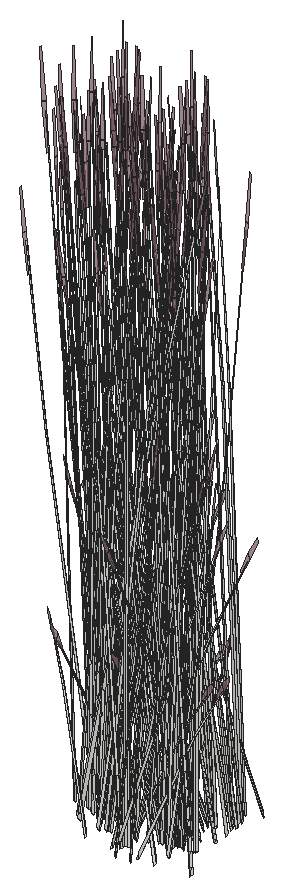
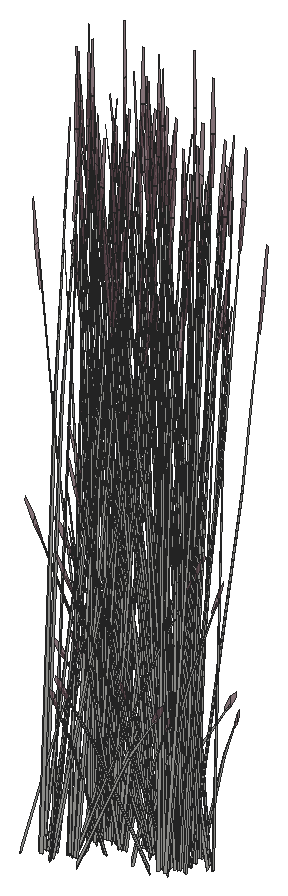
# SketchUp Ruby script. Lengths in inches.
U = 1.inch
M = Sketchup.active_model
def pt(a) = Geom::Point3d.new(a.map { |v| v * U })
def face(e, loops, mat)
  f = e.add_face(loops[0].map { |a| pt(a) })
  loops[1..].each { |l| e.add_face(l.map { |a| pt(a) }).erase! }
  f.material = f.back_material = mat if mat
  f
end
# faces: each face lists its corners as indices into pts; further lists are holes
def faces(e, pts, list, mat = nil) = list.each { |f| face(e, (f[0].is_a?(Array) ? f : [f]).map { |l| l.map { |i| pts[i] } }, mat) }
# xy, xz, yz: faces in a plane at the given z, y or x. An outline is a flat list of corners, or four numbers for a rectangle; further outlines are holes
def ring(l) = l.size == 4 ? [[l[0], l[1]], [l[2], l[1]], [l[2], l[3]], [l[0], l[3]]] : l.each_slice(2).to_a
def flat(e, list, mat, &to3) = list.each { |f| face(e, (f[0].is_a?(Array) ? f : [f]).map { |l| ring(l).map { |u, v| to3.(u, v) } }, mat) }
def xy(e, z, list, mat = nil) = flat(e, list, mat) { |x, y| [x, y, z] }
def xz(e, y, list, mat = nil) = flat(e, list, mat) { |x, z| [x, y, z] }
def yz(e, x, list, mat = nil) = flat(e, list, mat) { |y, z| [x, y, z] }
def lines(e, pts, list) = list.each { |a, b| e.add_line(pt(pts[a]), pt(pts[b])) }
# prism: a flat outline (further loops are holes) pulled along v
def prism(e, loops, v, mat = nil)
  f = face(e, loops, mat); d = Geom::Vector3d.new(v.map { |x| x * U })
  f.pushpull(f.normal.samedirection?(d) ? d.length : -d.length)
end
def box(e, o, s, mat = nil) = prism(e, [[o, [o[0] + s[0], o[1], o[2]], [o[0] + s[0], o[1] + s[1], o[2]], [o[0], o[1] + s[1], o[2]]]], [0, 0, s[2]], mat)
def at(x, y, z, deg = 0) = Geom::Transformation.translation(pt([x, y, z])) * Geom::Transformation.rotation(ORIGIN, Z_AXIS, deg.degrees)
def axes(o, x, y, z) = Geom::Transformation.new([*x, 0, *y, 0, *z, 0, *pt(o).to_a, 1])
def part(name) = M.definitions.add(name)
# library, detail: a bought-in or finely detailed component or shape, given as its bounding box
def library(name, o, s) = part(name).tap { |d| box(d.entities, o, s) }
def detail(e, o, s) = box(e.add_group.entities, o, s)
def put(e, d, t, mat = nil) = e.add_instance(d, t).tap { |i| i.material = mat if mat }
def group(e, t, mat = nil) = e.add_group.tap { |g| g.transformation = t; g.material = mat if mat }.entities
root = M.entities
M.materials.add("LightPink_Translucent").color = [144, 107, 117]
M.materials["LightPink_Translucent"].alpha = 0.75
c1 = part("blade")
p = [[2.15,0.21,22],[0,0.17,0],[0.09,0.45,0],[2.18,0.31,22],[2.29,0.31,22],[0.38,0.45,0],
  [2.48,0.24,33],[2.49,0.24,33],[2.48,0.22,33]]
faces(c1.entities,p,[[0,1,2,3],[4,5,2,3],[6,3,4,7],[8,0,3,6]])
c2 = part("seeds")
p = [[0.3,-0.1,1.38],[-0.01,-0.03,1.59],[-0.01,-0.03,0.03],[0.14,-0.07,-0.07],[0.29,-0.03,3],[0.15,0.01,3.11]]
faces(c2.entities,p,[[0,1,2,3],[1,0,4,5]],"LightPink_Translucent")
c3 = part("blade with seeds")
put(c3.entities,c1,at(0,0,0))
put(c3.entities,c2,axes([2.4,0.25,30.99],[1.5799,-0.05474,1.17369],[-0.12525,1.92788,0.29478],[-0.07173,-0.02425,1.56792]))
put(root,c3,axes([329.37,18.01,50.06],[0.63212,0.12701,0.27176],[-0.15814,0.45398,-0.32244],[-0.10462,0.05682,1.45692]))
put(root,c3,axes([329.32,18.31,49.78],[-0.47255,0.19538,-0.43871],[-0.28245,-0.35034,0],[-0.10763,0.0445,1.3917]))
put(root,c3,axes([334.98,18.31,49.78],[-0.47255,0.19538,-0.43871],[-0.28245,-0.35034,0],[-0.10763,0.0445,1.3917]))
put(root,c3,axes([330.85,20.33,50.4],[-0.24498,0.3521,0.39531],[-0.50902,-0.16945,-0.19025],[0,-0.08116,1.26923]))
put(root,c3,axes([330.89,17.16,49.78],[0,0.39075,-0.43871],[-0.56491,0,0],[0,0.089,1.3917]))
put(root,c3,axes([325.16,20.15,50.4],[-0.54829,0.02412,0.39531],[-0.04958,-0.40041,-0.19025],[0.09816,-0.04058,1.26923]))
put(root,c3,axes([331.75,20.02,49.95],[0,-0.45213,0],[0.63136,0,0],[0,0,1.58567]))
put(root,c3,axes([323.75,20.4375,50.19],[0,0.39075,0.43871],[-0.56491,0,0],[0,-0.089,1.3917]))
put(root,c3,axes([326.97,19.08,50.1],[0.31568,-0.39156,0],[0.52815,0.21836,-0.456],[0.12029,0.04973,1.44655]))
put(root,c3,axes([325.08,20.75,49.95],[-0.30332,-0.32798,-0.39531],[0.45944,-0.23096,0.19025],[-0.09816,-0.04058,1.26923]))
put(root,c3,axes([325.14,20.29,50.09],[0.21952,0.43694,0.40429],[-0.62724,0.15194,0.15865],[0.00767,-0.08029,1.40366]))
put(root,c3,axes([330.625,20.57,49.82],[-0.52523,-0.06406,-0.55095],[0.11084,-0.39517,-0.1446],[-0.15674,-0.04788,1.21613]))
put(root,c3,axes([331.45,19.74,50.09],[-0.41865,0.35461,0.40429],[-0.49737,-0.31303,0.15865],[0.10093,-0.03539,1.40366]))
put(root,c3,axes([328.21,20.625,49.75],[-0.3252,0.04689,1.25103],[-0.05176,-0.37326,0.07161],[0.22777,-0.0565,0.71188]))
put(root,c3,axes([328.8,20.3,50],[-0.31304,-0.24986,-0.05733],[0.34284,-0.22894,-0.25992],[0.09714,-0.01612,0.85731]))
put(root,c3,axes([331.91,20.37,50.03],[-0.46965,-0.33633,-0.05417],[0.46994,-0.33653,0],[-0.0164,-0.01174,1.55135]))
put(root,c3,axes([332.55,22.4,50.29],[-0.03058,0.12783,1.26356],[-0.44698,0.10701,-0.27174],[-0.10448,-0.16522,0.54024]))
put(root,c3,axes([325.03,20.64,50.4],[-0.24498,0.3521,0.39531],[-0.50902,-0.16945,-0.19025],[0,-0.08116,1.26923]))
put(root,c3,axes([330.72,19.15,50.1875],[-0.14586,0.38834,0.15589],[-0.53375,-0.1099,0.31002],[0.0922,-0.00189,1.41735]))
put(root,c3,axes([325.93,20.33,49.95],[0,-0.45213,0],[0.63136,0,0],[0,0,1.58567]))
put(root,c3,axes([326.7,19.28,50.19],[-0.47255,-0.19538,0.43871],[0.28245,-0.35034,0],[0.10763,0.0445,1.3917]))
put(root,c3,axes([329.75,18.25,50.1],[0.31568,0.39156,0],[-0.52815,0.21836,-0.456],[-0.12029,0.04973,1.44655]))
put(root,c3,axes([331.01,20.41,50.09],[0.63817,0.08233,0.40429],[-0.12987,0.46497,0.15865],[-0.09326,-0.0449,1.40366]))
put(root,c3,axes([330.25,18.39,49.32],[0.03679,-0.05641,1.55816],[0.46313,-0.16615,-0.23804],[0.14041,0.08599,0.26541]))
put(root,c3,axes([329.64,17.1,49.85],[0.18514,0.35777,-0.61156],[-0.53331,0.12885,-0.16051],[0.02046,0.12115,1.3499]))
put(root,c3,axes([325.63,20.04,50.09],[-0.41865,0.35461,0.40429],[-0.49737,-0.31303,0.15865],[0.10093,-0.03539,1.40366]))
put(root,c3,axes([326,18.34,49.32],[0.06773,0.03904,1.55816],[0.11484,0.36171,-0.23804],[-0.15011,0.07713,0.26541]))
put(root,c3,axes([331.66,18.34,49.32],[0.06773,0.03904,1.55816],[0.11484,0.36171,-0.23804],[-0.15011,0.07713,0.26541]))
put(root,c3,axes([328.94,20.01,49.32],[0.0128,0.06158,1.55816],[-0.25814,0.3216,-0.23804],[-0.18336,-0.01621,0.26541]))
put(root,c3,axes([331.63,19.68,50.4],[-0.30332,-0.32798,0.39531],[0.45944,-0.23096,-0.19025],[0.09816,0.04058,1.26923]))
put(root,c3,axes([326.09,20.68,50.03],[-0.46965,-0.33633,-0.05417],[0.46994,-0.33653,0],[-0.0164,-0.01174,1.55135]))
put(root,c3,axes([330.07,21.17,49.79],[-0.11861,-0.34048,-0.27372],[0.47106,-0.09668,0.27372],[-0.09497,-0.03926,1.22797]))
put(root,c3,axes([324.91,19.46,50.1875],[-0.14586,0.38834,0.15589],[-0.53375,-0.1099,0.31002],[0.0922,-0.00189,1.41735]))
put(root,c3,axes([324.68,19.77,49.41],[-0.49699,0.15644,1.13921],[-0.15819,-0.44887,0.44265],[0.30518,0.00747,1.29573]))
put(root,c3,axes([326.02,19.89,50.3125],[0.09741,-0.34873,0.12794],[0.4759,0.06053,-0.36534],[0.08661,0.03581,1.11991]))
put(root,c3,axes([330.67,21.15,50.1875],[0.54257,-0.10371,0.15589],[0.13397,0.38597,0.31002],[-0.04839,-0.05624,1.41735]))
put(root,c3,axes([330.22,18.48,50.36],[-0.32378,-0.01225,0.92831],[0.21383,-0.26028,0.51254],[0.12791,0.09247,0.72818]))
put(root,c3,axes([325.2,20.72,50.09],[0.63817,0.08233,0.40429],[-0.12987,0.46497,0.15865],[-0.09326,-0.0449,1.40366]))
put(root,c3,axes([328.57,20.38,49.32],[-0.02639,-0.05932,1.55816],[0.18302,-0.34702,-0.23804],[0.18462,-0.00499,0.26541]))
put(root,c3,axes([329.93,21.32,49.78],[-0.47255,-0.19538,-0.43871],[0.28245,-0.35034,0],[-0.10763,-0.0445,1.3917]))
put(root,c3,axes([325.82,19.98,50.4],[-0.30332,-0.32798,0.39531],[0.45944,-0.23096,-0.19025],[0.09816,0.04058,1.26923]))
put(root,c3,axes([332.18,20.12,49.95],[0.56491,0,0],[0,0.40454,0],[0,0,1.5764]))
put(root,c3,axes([331.22,20.63,50.36],[-0.50979,0.25942,-0.25709],[-0.339,-0.36656,-0.44182],[-0.12578,-0.03723,1.41118]))
put(root,c3,axes([332.34,19.17,50.1875],[-0.54257,0.10371,0.15589],[-0.13397,-0.38597,0.31002],[0.04839,0.05624,1.41735]))
put(root,c3,axes([324.85,21.46,50.1875],[0.54257,-0.10371,0.15589],[0.13397,0.38597,0.31002],[-0.04839,-0.05624,1.41735]))
put(root,c3,axes([325.97,20,50.36],[0.50979,-0.25942,-0.25709],[0.339,0.36656,-0.44182],[0.12578,0.03723,1.41118]))
put(root,c3,axes([329.16,17.85,50.29],[0.00891,-0.12953,1.26356],[0.4258,-0.14469,-0.27174],[0.13144,0.15503,0.54024]))
put(root,c3,axes([327.26,19.31,49.78],[0.47255,0.19538,-0.43871],[-0.28245,0.35034,0],[0.10763,0.0445,1.3917]))
put(root,c3,axes([326.36,20.43,49.95],[0.56491,0,0],[0,0.40454,0],[0,0,1.5764]))
put(root,c3,axes([331.99,19.92,50.1],[-0.63817,-0.08233,0.43472],[0.12987,-0.46497,0.17059],[0.09326,0.0449,1.50931]))
put(root,c3,axes([331.49,21.0625,49.95],[-0.16474,-0.33688,0],[0.47043,-0.11798,0],[0,0,1.36402]))
put(root,c3,axes([326.52,19.48,50.1875],[-0.54257,0.10371,0.15589],[-0.13397,-0.38597,0.31002],[0.04839,0.05624,1.41735]))
put(root,c3,axes([331.17,20.74,50.3125],[-0.09741,0.34873,0.12794],[-0.4759,-0.06053,-0.36534],[-0.08661,-0.03581,1.11991]))
put(root,c3,axes([332.29,21.18,50.1875],[0.14586,-0.38834,0.15589],[0.53375,0.1099,0.31002],[-0.0922,0.00189,1.41735]))
put(root,c3,axes([327.125,19.46,49.79],[0.11861,0.34048,-0.27372],[-0.47106,0.09668,0.27372],[0.09497,0.03926,1.22797]))
put(root,c3,axes([332.16,20.29,49.96],[0.35245,0.2524,0],[-0.35245,0.2524,0],[0,0,1.49564]))
put(root,c3,axes([328.09,18.375,49.32],[0.08172,-0.02126,1.55816],[0.49154,0.11703,-0.23804],[0.01437,0.1319,0.26541]))
put(root,c3,axes([333.12,20.18,50.1875],[-0.39671,-0.28463,0.15589],[0.39978,-0.27607,0.31002],[-0.04381,0.05813,1.41735]))
put(root,c3,axes([326.18,20.22,50.1],[-0.63817,-0.08233,0.43472],[0.12987,-0.46497,0.17059],[0.09326,0.0449,1.50931]))
put(root,c3,axes([325.67,21.37,49.95],[-0.16474,-0.33688,0],[0.47043,-0.11798,0],[0,0,1.36402]))
put(root,c3,axes([332.18,22.61,49.32],[-0.04891,0.05148,1.55816],[-0.49427,0.11098,-0.23804],[-0.1194,-0.10096,0.26541]))
put(root,c3,axes([331.37,21.22,49.94],[-0.50902,-0.17543,0],[0.24498,-0.36452,0],[0,0,1.43768]))
put(root,c3,axes([331.79,20.75,50.18],[-0.49304,-0.31451,-0.2226],[0.41487,-0.35316,0.48713],[-0.13277,0.03679,1.48635]))
put(root,c3,axes([325.35,21.05,50.3125],[-0.09741,0.34873,0.12794],[-0.4759,-0.06053,-0.36534],[-0.08661,-0.03581,1.11991]))
put(root,c3,axes([330.49,21.35,50.19],[0.47255,0.19538,0.43871],[-0.28245,0.35034,0],[-0.10763,-0.0445,1.3917]))
put(root,c3,axes([326.96,18.43,50.49],[0.45869,-0.0692,0.0575],[0.10545,0.27878,-0.76259],[-0.02908,0.14112,0.68355]))
put(root,c3,axes([332.62,18.43,50.49],[0.45869,-0.0692,0.0575],[0.10545,0.27878,-0.76259],[-0.02908,0.14112,0.68355]))
put(root,c3,axes([326.28,21.32,49.93],[0.53009,-0.13258,-0.16963],[0.18627,0.38191,0.00007],[0.05851,-0.01465,1.53656]))
put(root,c3,axes([333,24.02,49.85],[-0.20736,-0.4007,-0.61707],[0.59731,-0.14431,-0.16195],[-0.02292,-0.13569,1.36206]))
put(root,c3,axes([326.47,21.48,50.1875],[0.14586,-0.38834,0.15589],[0.53375,0.1099,0.31002],[-0.0922,0.00189,1.41735]))
put(root,c3,axes([332.16,20,50.4],[0.24498,-0.3521,0.39531],[0.50902,0.16945,-0.19025],[0,0.08116,1.26923]))
put(root,c3,axes([326.35,20.6,49.96],[0.35245,0.2524,0],[-0.35245,0.2524,0],[0,0,1.49564]))
put(root,c3,axes([327.3,20.49,50.1875],[-0.39671,-0.28463,0.15589],[0.39978,-0.27607,0.31002],[-0.04381,0.05813,1.41735]))
put(root,c3,axes([326.57,20.0625,49.82],[0.52523,0.06406,-0.55095],[-0.11084,0.39517,-0.1446],[0.15674,0.04788,1.21613]))
put(root,c3,axes([332.07,20.2,50.03],[0,0.45191,-0.04981],[-0.63136,0,0],[0,0.0142,1.58489]))
put(root,c3,axes([330.22,21.56,50.1],[-0.31568,0.39156,0],[-0.52815,-0.21836,-0.456],[-0.12029,-0.04973,1.44655]))
put(root,c3,axes([325.55,21.52,49.94],[-0.50902,-0.17543,0],[0.24498,-0.36452,0],[0,0,1.43768]))
put(root,c3,axes([325.97,21.06,50.18],[-0.49304,-0.31451,-0.2226],[0.41487,-0.35316,0.48713],[-0.13277,0.03679,1.48635]))
put(root,c3,axes([324.68,21.66,50.19],[0.47255,0.19538,0.43871],[-0.28245,0.35034,0],[-0.10763,-0.0445,1.3917]))
put(root,c3,axes([332.03,20.49,50.4],[0.54829,-0.02412,0.39531],[0.04958,0.40041,-0.19025],[-0.09816,0.04058,1.26923]))
put(root,c3,axes([326.34,20.31,50.4],[0.24498,-0.3521,0.39531],[0.50902,0.16945,-0.19025],[0,0.08116,1.26923]))
put(root,c3,axes([331.54,20.68,49.95],[-0.54829,0.02412,-0.39531],[-0.04958,-0.40041,0.19025],[-0.09816,0.04058,1.26923]))
put(root,c3,axes([333.61,22.4,49.88],[-0.34892,0.22417,-0.0344],[-0.3197,-0.24551,-0.15595],[-0.02251,-0.06957,0.51438]))
put(root,c3,axes([326.25,20.51,50.03],[0,0.45191,-0.04981],[-0.63136,0,0],[0,0.0142,1.58489]))
put(root,c3,axes([326.29,20.1875,49.95],[0.30332,0.32798,-0.39531],[-0.45944,0.23096,0.19025],[0.09816,0.04058,1.26923]))
put(root,c3,axes([331.95,21.22,49.95],[0.50902,0.17543,0],[-0.24498,0.36452,0],[0,0,1.54589]))
put(root,c3,axes([327.63,20.5,50.19],[0,-0.39075,0.43871],[0.56491,0,0],[0,0.089,1.3917]))
put(root,c3,axes([326.21,20.8,50.4],[0.54829,-0.02412,0.39531],[0.04958,0.40041,-0.19025],[-0.09816,0.04058,1.26923]))
put(root,c3,axes([326.85,18.72,50.29],[0.15933,-0.06164,1.26356],[0.39339,0.18587,-0.27174],[-0.11709,0.16083,0.54024]))
put(root,c3,axes([332.51,18.72,50.29],[0.15933,-0.06164,1.26356],[0.39339,0.18587,-0.27174],[-0.11709,0.16083,0.54024]))
put(root,c3,axes([326.56,20.39,50.3125],[0.47043,-0.11396,0.12794],[0.16474,0.32541,-0.36534],[0,0.07162,1.11991]))
put(root,c3,axes([332.15,21.61,49.9375],[-0.31175,-0.39292,-0.04544],[0.52815,-0.21836,0.456],[-0.13015,0.03741,1.44584]))
put(root,c3,axes([325.73,20.99,49.95],[-0.54829,0.02412,-0.39531],[-0.04958,-0.40041,0.19025],[-0.09816,0.04058,1.26923]))
put(root,c3,axes([332.04,20.66,50.3125],[0.37303,0.23477,0.12794],[-0.31115,0.26487,-0.36534],[-0.08661,0.03581,1.11991]))
put(root,c3,axes([328.3,21.18,50.29],[-0.1216,-0.0961,1.26356],[0.15822,-0.31792,-0.27174],[0.24603,0.04307,0.54024]))
put(root,c3,axes([331.78,23.97,49.78],[0,-0.39075,-0.43871],[0.56491,0,0],[0,-0.089,1.3917]))
put(root,c3,axes([326.13,21.53,49.95],[0.50902,0.17543,0],[-0.24498,0.36452,0],[0,0,1.54589]))
put(root,c3,axes([332.4375,21.38,50.19],[0.47255,-0.19538,0.43871],[0.28245,0.35034,0],[-0.10763,0.0445,1.3917]))
put(root,c3,axes([326.33,21.92,49.9375],[-0.31175,-0.39292,-0.04544],[0.52815,-0.21836,0.456],[-0.13015,0.03741,1.44584]))
put(root,c3,axes([326.22,20.97,50.3125],[0.37303,0.23477,0.12794],[-0.31115,0.26487,-0.36534],[-0.08661,0.03581,1.11991]))
put(root,c3,axes([331.76,21.08,50.02],[0.21952,0.44891,-0.05313],[-0.62724,0.1573,0],[0.00767,0.01568,1.52132]))
put(root,c3,axes([332.01,21.5625,49.79],[-0.47106,-0.09668,-0.27372],[0.11861,-0.34048,0.27372],[-0.09497,0.03926,1.22797]))
put(root,c3,axes([328.61,20.87,50.29],[0.17547,0.03208,1.26356],[0.1131,0.32764,-0.27174],[-0.23835,0.06133,0.54024]))
put(root,c3,axes([333.58,20.49,49.94],[-0.63105,-0.00312,-0.04397],[0,-0.43672,0.44129],[-0.01983,0.09942,1.3992]))
put(root,c3,axes([332.02,23.97,49.79],[0.35245,-0.2438,-0.27372],[0.35245,0.2438,0.27372],[0,-0.07853,1.22797]))
put(root,c3,axes([333.45,20.55,49.79],[-0.35245,0.2438,-0.27372],[-0.35245,-0.2438,0.27372],[0,0.07853,1.22797]))
put(root,c3,axes([326.62,21.69,50.19],[0.47255,-0.19538,0.43871],[0.28245,0.35034,0],[-0.10763,0.0445,1.3917]))
put(root,c3,axes([331.93,20.57,50.36],[0.05884,0.44587,-0.25709],[-0.6128,0.02696,-0.44182],[-0.10791,0.05939,1.41118]))
put(root,c3,axes([331.88,22.81,49.88],[-0.14565,0.31907,-0.0344],[-0.44829,-0.09815,-0.15595],[-0.06806,-0.05219,0.51438]))
put(root,c3,axes([333.25,24.42,50.36],[-0.56863,-0.18645,-0.25709],[0.2738,-0.39352,-0.44182],[-0.01787,-0.09662,1.41118]))
put(root,c3,axes([332.15,20.4,49.95],[-0.24498,0.3521,-0.39531],[-0.50902,-0.16945,0.19025],[0,0.08116,1.26923]))
put(root,c3,axes([325.95,21.38,50.02],[0.21952,0.44891,-0.05313],[-0.62724,0.1573,0],[0.00767,0.01568,1.52132]))
put(root,c3,axes([326.19,21.87,49.79],[-0.47106,-0.09668,-0.27372],[0.11861,-0.34048,0.27372],[-0.09497,0.03926,1.22797]))
put(root,c3,axes([331.64,24.26,50.1],[-0.63136,0,0],[0,-0.43672,-0.456],[0,-0.09947,1.44655]))
put(root,c3,axes([331.74,23.48,50.29],[0.09858,0.10879,1.26356],[-0.22716,0.29571,-0.27174],[-0.23325,-0.07068,0.54024]))
put(root,c3,axes([328.01,20.57,50.1],[0.63136,0,0],[0,0.43672,-0.456],[0,0.09947,1.44655]))
put(root,c3,axes([327.76,20.79,49.94],[-0.63105,-0.00312,-0.04397],[0,-0.43672,0.44129],[-0.01983,0.09942,1.3992]))
put(root,c3,axes([326.39,20.41,50.36],[0.56863,0.18645,-0.25709],[-0.2738,0.39352,-0.44182],[0.01787,0.09662,1.41118]))
put(root,c3,axes([327.63,20.86,49.79],[-0.35245,0.2438,-0.27372],[-0.35245,-0.2438,0.27372],[0,0.07853,1.22797]))
put(root,c3,axes([326.11,20.88,50.36],[0.05884,0.44587,-0.25709],[-0.6128,0.02696,-0.44182],[-0.10791,0.05939,1.41118]))
put(root,c3,axes([331.56,20.91,49.82],[-0.34009,0.2937,-0.55095],[-0.42248,-0.26632,-0.1446],[-0.13628,0.07327,1.21613]))
put(root,c3,axes([326.33,20.71,49.95],[-0.24498,0.3521,-0.39531],[-0.50902,-0.16945,0.19025],[0,0.08116,1.26923]))
put(root,c3,axes([332.16,21.41,50.06],[0.63212,0.12701,0.27176],[-0.15814,0.45398,-0.32244],[-0.10462,0.05682,1.45692]))
put(root,c3,axes([332.12,21.72,49.78],[-0.47255,0.19538,-0.43871],[-0.28245,-0.35034,0],[-0.10763,0.0445,1.3917]))
put(root,c3,axes([332.125,24.15,50.06],[-0.46965,0.32852,0.27176],[-0.46994,-0.32506,-0.32244],[-0.0164,-0.09329,1.45692]))
put(root,c3,axes([326.35,21.72,50.06],[0.63212,0.12701,0.27176],[-0.15814,0.45398,-0.32244],[-0.10462,0.05682,1.45692]))
put(root,c3,axes([333.4,24.83,50.16],[0.13383,-0.46302,-0.20702],[0.63453,0.08071,0.45303],[-0.11087,-0.06394,1.38231]))
put(root,c3,axes([326.3,22.02,49.78],[-0.47255,0.19538,-0.43871],[-0.28245,-0.35034,0],[-0.10763,0.0445,1.3917]))
put(root,c3,axes([327.87,20.87,49.78],[0,0.39075,-0.43871],[-0.56491,0,0],[0,0.089,1.3917]))
put(root,c3,axes([332.55,21.65,50.1],[0.31568,0.39156,0],[-0.52815,0.21836,-0.456],[-0.12029,0.04973,1.44655]))
put(root,c3,axes([332.4375,20.51,49.85],[0.18514,0.35777,-0.61156],[-0.53331,0.12885,-0.16051],[0.02046,0.12115,1.3499]))
put(root,c3,axes([328.8,21.74,49.32],[0.06773,0.03904,1.55816],[0.11484,0.36171,-0.23804],[-0.15011,0.07713,0.26541]))
put(root,c3,axes([332.02,24.33,50.19],[0,0.39075,0.43871],[-0.56491,0,0],[0,-0.089,1.3917]))
put(root,c3,axes([333.35,24.64,49.95],[-0.30332,-0.32798,-0.39531],[0.45944,-0.23096,0.19025],[-0.09816,-0.04058,1.26923]))
put(root,c3,axes([334.39,26.18,50.29],[-0.03058,0.12783,1.26356],[-0.44698,0.10701,-0.27174],[-0.10448,-0.16522,0.54024]))
put(root,c3,axes([326.73,21.96,50.1],[0.31568,0.39156,0],[-0.52815,0.21836,-0.456],[-0.12029,0.04973,1.44655]))
put(root,c3,axes([333.31,24.52,50.4],[-0.24498,0.3521,0.39531],[-0.50902,-0.16945,-0.19025],[0,-0.08116,1.26923]))
put(root,c3,axes([327.23,22.09,49.32],[0.03679,-0.05641,1.55816],[0.46313,-0.16615,-0.23804],[0.14041,0.08599,0.26541]))
put(root,c3,axes([326.62,20.8125,49.85],[0.18514,0.35777,-0.61156],[-0.53331,0.12885,-0.16051],[0.02046,0.12115,1.3499]))
put(root,c3,axes([333.08,24.77,49.82],[-0.52523,-0.06406,-0.55095],[0.11084,-0.39517,-0.1446],[-0.15674,-0.04788,1.21613]))
put(root,c3,axes([327.2,22.1875,50.36],[-0.32378,-0.01225,0.92831],[0.21383,-0.26028,0.51254],[0.12791,0.09247,0.72818]))
put(root,c3,axes([333.47,24.61,50.09],[0.63817,0.08233,0.40429],[-0.12987,0.46497,0.15865],[-0.09326,-0.0449,1.40366]))
put(root,c3,axes([331.39,24.21,49.32],[0.0128,0.06158,1.55816],[-0.25814,0.3216,-0.23804],[-0.18336,-0.01621,0.26541]))
put(root,c3,axes([326.14,21.56,50.29],[0.00891,-0.12953,1.26356],[0.4258,-0.14469,-0.27174],[0.13144,0.15503,0.54024]))
put(root,c3,axes([332.52,25.37,49.79],[-0.11861,-0.34048,-0.27372],[0.47106,-0.09668,0.27372],[-0.09497,-0.03926,1.22797]))
put(root,c3,axes([330.89,21.77,49.32],[0.08172,-0.02126,1.55816],[0.49154,0.11703,-0.23804],[0.01437,0.1319,0.26541]))
put(root,c3,axes([333.13,25.35,50.1875],[0.54257,-0.10371,0.15589],[0.13397,0.38597,0.31002],[-0.04839,-0.05624,1.41735]))
put(root,c3,axes([329.76,21.83,50.49],[0.45869,-0.0692,0.0575],[0.10545,0.27878,-0.76259],[-0.02908,0.14112,0.68355]))
